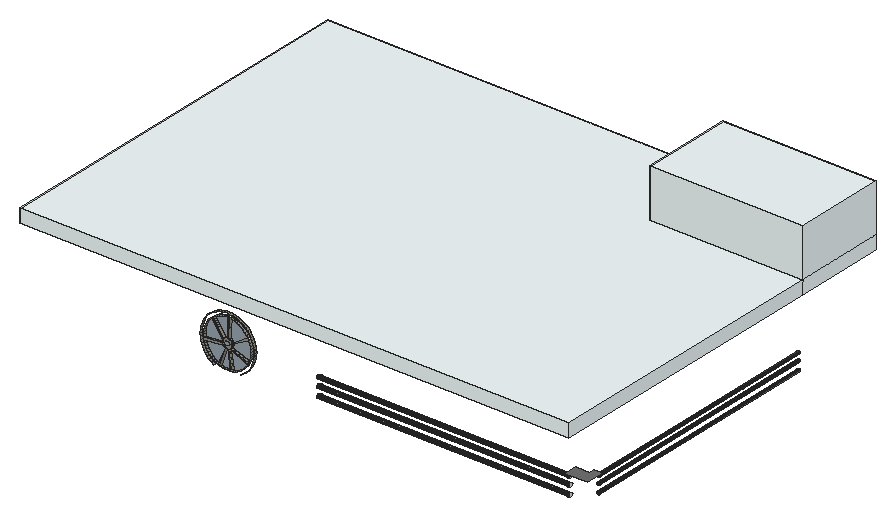
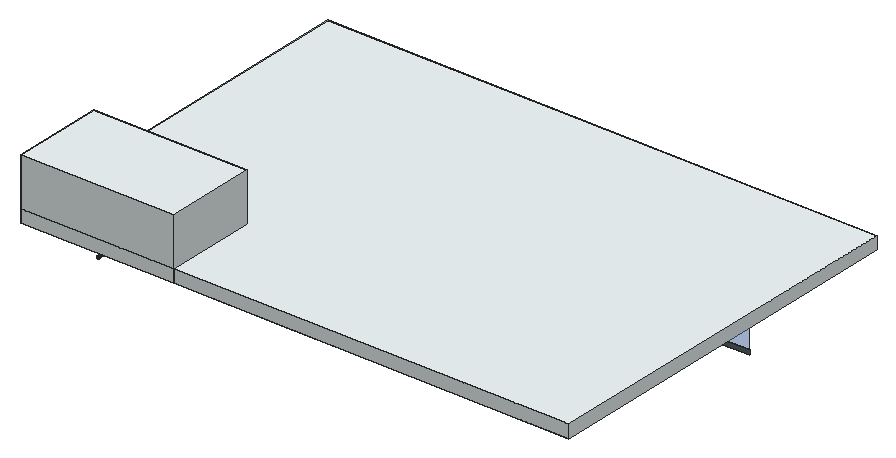
# SketchUp Ruby script. Lengths in inches.
U = 1.inch
M = Sketchup.active_model
def pt(a) = Geom::Point3d.new(a.map { |v| v * U })
def face(e, loops, mat)
  f = e.add_face(loops[0].map { |a| pt(a) })
  loops[1..].each { |l| e.add_face(l.map { |a| pt(a) }).erase! }
  f.material = f.back_material = mat if mat
  f
end
# faces: each face lists its corners as indices into pts; further lists are holes
def faces(e, pts, list, mat = nil) = list.each { |f| face(e, (f[0].is_a?(Array) ? f : [f]).map { |l| l.map { |i| pts[i] } }, mat) }
# xy, xz, yz: faces in a plane at the given z, y or x. An outline is a flat list of corners, or four numbers for a rectangle; further outlines are holes
def ring(l) = l.size == 4 ? [[l[0], l[1]], [l[2], l[1]], [l[2], l[3]], [l[0], l[3]]] : l.each_slice(2).to_a
def flat(e, list, mat, &to3) = list.each { |f| face(e, (f[0].is_a?(Array) ? f : [f]).map { |l| ring(l).map { |u, v| to3.(u, v) } }, mat) }
def xy(e, z, list, mat = nil) = flat(e, list, mat) { |x, y| [x, y, z] }
def xz(e, y, list, mat = nil) = flat(e, list, mat) { |x, z| [x, y, z] }
def yz(e, x, list, mat = nil) = flat(e, list, mat) { |y, z| [x, y, z] }
def lines(e, pts, list) = list.each { |a, b| e.add_line(pt(pts[a]), pt(pts[b])) }
# prism: a flat outline (further loops are holes) pulled along v
def prism(e, loops, v, mat = nil)
  f = face(e, loops, mat); d = Geom::Vector3d.new(v.map { |x| x * U })
  f.pushpull(f.normal.samedirection?(d) ? d.length : -d.length)
end
def box(e, o, s, mat = nil) = prism(e, [[o, [o[0] + s[0], o[1], o[2]], [o[0] + s[0], o[1] + s[1], o[2]], [o[0], o[1] + s[1], o[2]]]], [0, 0, s[2]], mat)
def at(x, y, z, deg = 0) = Geom::Transformation.translation(pt([x, y, z])) * Geom::Transformation.rotation(ORIGIN, Z_AXIS, deg.degrees)
def axes(o, x, y, z) = Geom::Transformation.new([*x, 0, *y, 0, *z, 0, *pt(o).to_a, 1])
def part(name) = M.definitions.add(name)
# library, detail: a bought-in or finely detailed component or shape, given as its bounding box
def library(name, o, s) = part(name).tap { |d| box(d.entities, o, s) }
def detail(e, o, s) = box(e.add_group.entities, o, s)
def put(e, d, t, mat = nil) = e.add_instance(d, t).tap { |i| i.material = mat if mat }
def group(e, t, mat = nil) = e.add_group.tap { |g| g.transformation = t; g.material = mat if mat }.entities
root = M.entities
M.materials.add("[Color M04]").color = [142, 142, 142]
M.materials.add("[Color M05]").color = [114, 114, 114]
M.materials.add("[Formica Graystone]1").color = [149, 146, 135]
M.materials.add("[Formica Speckled Grey]").color = [94, 105, 111]
M.materials.add("[Terrazzo Light Blue]").color = [151, 165, 175]
M.materials.add("[Terrazzo Light Blue]1").color = [196, 214, 227]
M.materials.add("[Translucent Glass Blue]").color = [100, 149, 237]
M.materials["[Translucent Glass Blue]"].alpha = 0.5
M.materials.add("[White Subway Tile]").color = [243, 252, 253]
xy(root,2160.625,[[2109.83,824.72,2111.95,824.99,2113.93,825.8125,2115.625,827.11,2116.92,828.81,2117.74,830.78,2118.02,832.9,2117.74,835.02,2116.92,837,2115.625,838.69,2113.93,839.99,2111.95,840.8125,2109.83,841.09,2107.72,840.8125,2105.74,839.99,2104.04,838.69,2102.74,837,2101.93,835.02,2101.65,832.9,2101.93,830.78,2102.74,828.81,2104.04,827.11,2105.74,825.8125,2107.72,824.99]])
xy(root,2167.3125,[[2949.99,1696.19,2952.05,1696.46,2953.96,1697.25,2955.6,1698.51,2956.87,1700.16,2957.66,1702.07,2957.93,1704.13,2957.66,1706.18,2956.87,1708.1,2955.6,1709.74,2953.96,1711,2952.05,1711.79,2949.99,1712.06,2947.9375,1711.79,2946.02,1711,2944.38,1709.74,2943.12,1708.1,2942.32,1706.18,2942.05,1704.13,2942.32,1702.07,2943.12,1700.16,2944.38,1698.51,2946.02,1697.25,2947.9375,1696.46]])
xy(root,2167.625,[[2949.99,1302.69,2952.05,1302.96,2953.96,1303.75,2955.6,1305.01,2956.87,1306.66,2957.66,1308.57,2957.93,1310.63,2957.66,1312.68,2956.87,1314.6,2955.6,1316.24,2953.96,1317.5,2952.05,1318.29,2949.99,1318.56,2947.9375,1318.29,2946.02,1317.5,2944.38,1316.24,2943.12,1314.6,2942.32,1312.68,2942.05,1310.63,2942.32,1308.57,2943.12,1306.66,2944.38,1305.01,2946.02,1303.75,2947.9375,1302.96]])
xy(root,2183.75,[[2867.16,803.71,2968.68,803.71,2968.68,888.17,2929.99,888.17,2929.99,862.88,2867.16,862.88]],"[Color M05]")
xy(root,2330.11,[[1687.83,876.99,1720.33,1103.3]],"[Terrazzo Light Blue]")
xy(root,2340.5,[[605.8,1146.14,928.48,1221.7]])
xy(root,2410.6875,[[477.43,697.64,547.35,1118.14],[2764.79,697.64,2968.68,2026.57],[1034.97,803.71,1720.33,2026.57],[477.43,1118.14,547.35,1118.14,547.35,1146.14,1034.97,1146.14,1034.97,2026.57,477.43,2026.57],[1720.33,1239.01,2764.79,2026.57],
  [477.43,2026.57,1034.97,2442.87],[1034.97,2026.57,1720.33,2442.87],[1720.33,2026.57,2273.77,2442.87],[2273.77,2026.57,2968.68,2442.87]])
xy(root,2410.6875,[[547.35,697.64,1034.97,1146.14],[1034.97,697.64,1720.33,803.71],[[1720.33,697.64,2764.79,1239.01],[2267.4,882.09,2324.97,939.65]]],"[Terrazzo Light Blue]1")
xy(root,2470.25,[[477.43,697.64,2968.68,2442.87]],"[White Subway Tile]")
xy(root,2688.875,[[2273.77,2026.57,2968.68,2442.87]],"[White Subway Tile]")
xz(root,697.64,[[477.43,2410.6875,2968.68,2470.25]],"[White Subway Tile]")
xz(root,793.39,[[1352.48,2073.62,1363.66,2075.39,1346.76,2160.28],[1307.78,2078.32,1335.6,2160.28,1297.22,2082.37],[1434.79,2127.07,1439.92,2137.15,1356.43,2165.86],[1235.46,2158.64,1322.51,2170.33,1320.36,2175.53,1233.69,2169.8125],[[1341.18,2159.55,1346.76,2160.28,1351.96,2162.4375,1356.43,2165.86,1359.86,2170.33,1362.01,2175.53,1362.75,2181.11,1362.01,2186.69,1359.86,2191.89,1356.43,2196.36,1351.96,2199.79,1346.76,2201.94,1341.18,2202.67,1335.6,2201.94,1330.4,2199.79,1325.9375,2196.36,1322.51,2191.89,1320.36,2186.69,1319.62,2181.11,1320.36,2175.53,1322.51,2170.33,1325.9375,2165.86,1330.4,2162.4375,1335.6,2160.28],[1341.86,2170.07,1339.11,2170.1,1336.45,2170.84,1334.08,2172.24,1332.15,2174.21,1330.79,2176.62,1330.11,2179.29,1330.14,2182.04,1330.88,2184.7,1332.28,2187.07,1334.25,2189,1336.65,2190.36,1339.32,2191.04,1342.08,2191.02,1344.74,2190.27,1347.11,2188.87,1349.04,2186.9,1350.39,2184.5,1351.08,2181.83,1351.05,2179.07,1350.31,2176.42,1348.91,2174.04,1346.9375,2172.11,1344.54,2170.76]],
  [1362.01,2186.69,1439.92,2225.07,1434.79,2235.15],[1322.51,2191.89,1325.9375,2196.36,1277.65,2268.55,1268.86,2261.43],[1346.76,2201.94,1352.48,2288.6,1341.18,2289.2,1341.18,2202.67]],"[Formica Graystone]1")
xz(root,793.39,[[1341.86,2170.07,1344.54,2170.76,1346.9375,2172.11,1348.91,2174.04,1350.31,2176.42,1351.05,2179.07,1351.08,2181.83,1350.39,2184.5,1349.04,2186.9,1347.11,2188.87,1344.74,2190.27,1342.08,2191.02,1339.32,2191.04,1336.65,2190.36,1334.25,2189,1332.28,2187.07,1330.88,2184.7,1330.14,2182.04,1330.11,2179.29,1330.79,2176.62,1332.15,2174.21,1334.08,2172.24,1336.45,2170.84,1339.11,2170.1]],"[Terrazzo Light Blue]")
xz(root,803.71,[[1341.18,2073.03,1352.48,2073.62,1346.76,2160.28,1341.18,2159.55,1335.6,2160.28,1307.78,2078.32,1318.71,2075.39,1329.89,2073.62],[1363.66,2075.39,1374.58,2078.32,1385.15,2082.37,1395.23,2087.51,1404.71,2093.67,1413.51,2100.79,1421.51,2108.79,1428.625,2117.58,1434.79,2127.07,1356.43,2165.86,1351.96,2162.4375,1346.76,2160.28],[1297.22,2082.37,1335.6,2160.28,1330.4,2162.4375,1325.9375,2165.86,1322.51,2170.33,1235.46,2158.64,1238.39,2147.71,1242.44,2137.15,1247.58,2127.07,1253.74,2117.58,1260.86,2108.79,1268.86,2100.79,1277.65,2093.67,1287.14,2087.51],[1439.92,2137.15,1443.98,2147.71,1446.91,2158.64,1448.68,2169.8125,1449.27,2181.11,1448.68,2192.41,1446.91,2203.58,1443.98,2214.51,1439.92,2225.07,1362.01,2186.69,1362.75,2181.11,1362.01,2175.53,1359.86,2170.33,1356.43,2165.86],[1233.69,2169.8125,1320.36,2175.53,1319.62,2181.11,1320.36,2186.69,1322.51,2191.89,1268.86,2261.43,1260.86,2253.43,1253.74,2244.64,1247.58,2235.15,1242.44,2225.07,1238.39,2214.51,1235.46,2203.58,1233.69,2192.41,1233.1,2181.11],
  [1362.01,2186.69,1434.79,2235.15,1428.625,2244.64,1421.51,2253.43,1413.51,2261.43,1404.71,2268.55,1395.23,2274.72,1385.15,2279.85,1374.58,2283.91,1363.66,2286.84,1352.48,2288.6,1346.76,2201.94,1351.96,2199.79,1356.43,2196.36,1359.86,2191.89],[1325.9375,2196.36,1330.4,2199.79,1335.6,2201.94,1341.18,2202.67,1341.18,2289.2,1329.89,2288.6,1318.71,2286.84,1307.78,2283.91,1297.22,2279.85,1287.14,2274.72,1277.65,2268.55]],"[Terrazzo Light Blue]")
xz(root,888.17,[[2950.45,2090.97,2952.01,2091.18,2953.45,2091.77,2954.7,2092.73,2955.65,2093.97,2956.25,2095.42,2956.45,2096.97,2956.25,2098.52,2955.65,2099.97,2954.7,2101.21,2953.45,2102.17,2952.01,2102.77,2950.45,2102.97,2948.9,2102.77,2947.45,2102.17,2946.21,2101.21,2945.26,2099.97,2944.66,2098.52,2944.45,2096.97,2944.66,2095.42,2945.26,2093.97,2946.21,2092.73,2947.45,2091.77,2948.9,2091.18],[2950.45,2128.53,2952.01,2128.74,2953.45,2129.34,2954.7,2130.29,2955.65,2131.53,2956.25,2132.98,2956.45,2134.53,2956.25,2136.09,2955.65,2137.53,2954.7,2138.78,2953.45,2139.73,2952.01,2140.33,2950.45,2140.53,2948.9,2140.33,2947.45,2139.73,2946.21,2138.78,2945.26,2137.53,2944.66,2136.09,2944.45,2134.53,2944.66,2132.98,2945.26,2131.53,2946.21,2130.29,2947.45,2129.34,2948.9,2128.74],[2950.45,2161.72,2952.01,2161.93,2953.45,2162.52,2954.7,2163.48,2955.65,2164.72,2956.25,2166.17,2956.45,2167.72,2956.25,2169.27,2955.65,2170.72,2954.7,2171.96,2953.45,2172.92,2952.01,2173.52,2950.45,2173.72,2948.9,2173.52,2947.45,2172.92,2946.21,2171.96,2945.26,2170.72,2944.66,2169.27,2944.45,2167.72,2944.66,2166.17,2945.26,2164.72,2946.21,2163.48,2947.45,2162.52,2948.9,2161.93]])
xz(root,1221.7,[[631.45,2158.7,755.72,2178.96],[755.72,2158.7,770.95,2178.96],[770.95,2158.7,902.82,2178.96],[755.72,2178.96,770.95,2314.84]],"[Formica Speckled Grey]")
xz(root,1221.7,[[631.45,2178.96,755.72,2314.84],[770.95,2178.96,902.82,2314.84]],"[Translucent Glass Blue]")
xz(root,2026.57,[[2273.77,2410.6875,2968.68,2688.875]],"[White Subway Tile]")
xz(root,2442.87,[[477.43,2410.6875,2273.77,2470.25],[2273.77,2410.6875,2968.68,2470.25],[2273.77,2470.25,2968.68,2688.875]],"[White Subway Tile]")
yz(root,477.43,[[697.64,2410.6875,2442.87,2470.25]],"[White Subway Tile]")
yz(root,1341.18,[[793.39,2202.67,803.71,2289.2]],"[Formica Graystone]1")
yz(root,2273.77,[[2026.57,2410.6875,2442.87,2688.875]],"[White Subway Tile]")
yz(root,2867.16,[[836.16,2075.23,838.2,2075.5,840.1,2076.28,841.73,2077.53,842.98,2079.16,843.77,2081.0625,844.04,2083.1,843.77,2085.14,842.98,2087.04,841.73,2088.67,840.1,2089.92,838.2,2090.71,836.16,2090.98,834.125,2090.71,832.22,2089.92,830.59,2088.67,829.34,2087.04,828.55,2085.14,828.29,2083.1,828.55,2081.0625,829.34,2079.16,830.59,2077.53,832.22,2076.28,834.125,2075.5],[836.16,2115.79,838.2,2116.06,840.1,2116.84,841.73,2118.1,842.98,2119.73,843.77,2121.625,844.04,2123.66,843.77,2125.7,842.98,2127.6,841.73,2129.23,840.1,2130.48,838.2,2131.27,836.16,2131.54,834.125,2131.27,832.22,2130.48,830.59,2129.23,829.34,2127.6,828.55,2125.7,828.29,2123.66,828.55,2121.625,829.34,2119.73,830.59,2118.1,832.22,2116.84,834.125,2116.06],[836.16,2153.1,838.2,2153.37,840.1,2154.16,841.73,2155.41,842.98,2157.04,843.77,2158.9375,844.04,2160.98,843.77,2163.02,842.98,2164.91,841.73,2166.55,840.1,2167.8,838.2,2168.58,836.16,2168.85,834.125,2168.58,832.22,2167.8,830.59,2166.55,829.34,2164.91,828.55,2163.02,828.29,2160.98,828.55,2158.9375,829.34,2157.04,830.59,2155.41,832.22,2154.16,834.125,2153.37]])
yz(root,2968.68,[[697.64,2410.6875,2026.57,2470.25],[2026.57,2410.6875,2442.87,2470.25],[2026.57,2470.25,2442.87,2688.875]],"[White Subway Tile]")
p = [[1341.18,803.71,2073.03],[1329.89,803.71,2073.62],[1329.89,793.39,2073.62],[1341.18,793.39,2073.03],[1352.48,803.71,2073.62],[1352.48,793.39,2073.62],
  [1318.71,803.71,2075.39],[1318.71,793.39,2075.39],[1346.76,803.71,2160.28],[1346.76,793.39,2160.28],[1268.59,803.71,2081.2],[1279.43,803.71,2074.16],
  [1279.43,793.39,2074.16],[1268.59,793.39,2081.2],[1402.93,803.71,2074.16],[1413.77,803.71,2081.2],[1413.77,793.39,2081.2],[1402.93,793.39,2074.16],
  [2867.16,836.16,2075.23],[2867.16,834.125,2075.5],[1720.33,834.125,2075.5],[1720.33,836.16,2075.23],[2867.16,838.2,2075.5],[1720.33,838.2,2075.5],
  [1307.78,803.71,2078.32],[1307.78,793.39,2078.32],[1363.66,803.71,2075.39],[1363.66,793.39,2075.39],[1374.58,803.71,2078.32],[1374.58,793.39,2078.32],
  [2867.16,832.22,2076.28],[1720.33,832.22,2076.28],[2867.16,840.1,2076.28],[1720.33,840.1,2076.28],[2867.16,830.59,2077.53],[1720.33,830.59,2077.53],
  [2867.16,841.73,2077.53],[1720.33,841.73,2077.53],[2867.16,829.34,2079.16],[1720.33,829.34,2079.16],[2867.16,842.98,2079.16],[1720.33,842.98,2079.16],
  [1335.6,803.71,2160.28],[1335.6,793.39,2160.28],[1385.15,803.71,2082.37],[1385.15,793.39,2082.37],[2867.16,828.55,2081.0625],[1720.33,828.55,2081.0625],
  [2867.16,843.77,2081.0625],[1720.33,843.77,2081.0625],[2867.16,828.29,2083.1],[1720.33,828.29,2083.1],[2867.16,844.04,2083.1],[1720.33,844.04,2083.1],
  [1258.55,803.71,2089.33],[1258.55,793.39,2089.33],[1423.82,803.71,2089.33],[1423.82,793.39,2089.33],[1297.22,803.71,2082.37],[1287.14,803.71,2087.51],
  [1287.14,793.39,2087.51],[1297.22,793.39,2082.37],[1395.23,803.71,2087.51],[1395.23,793.39,2087.51],[2867.16,828.55,2085.14],[1720.33,828.55,2085.14],
  [2867.16,843.77,2085.14],[1720.33,843.77,2085.14],[2867.16,829.34,2087.04],[1720.33,829.34,2087.04],[2867.16,842.98,2087.04],[1720.33,842.98,2087.04],
  [2867.16,830.59,2088.67],[1720.33,830.59,2088.67],[2867.16,841.73,2088.67],[1720.33,841.73,2088.67],[1277.65,803.71,2093.67],[1277.65,793.39,2093.67],
  [1404.71,803.71,2093.67],[1404.71,793.39,2093.67],[2867.16,832.22,2089.92],[1720.33,832.22,2089.92],[2867.16,840.1,2089.92],[1720.33,840.1,2089.92],
  [1249.4,803.71,2098.47],[1249.4,793.39,2098.47],[1432.96,803.71,2098.47],[1432.96,793.39,2098.47],[2867.16,834.125,2090.71],[1720.33,834.125,2090.71],
  [2867.16,838.2,2090.71],[1720.33,838.2,2090.71],[2867.16,836.16,2090.98],[1720.33,836.16,2090.98],[2950.45,888.17,2090.97],[2948.9,888.17,2091.18],
  [2948.9,2026.57,2091.18],[2950.45,2026.57,2090.97],[2952.01,888.17,2091.18],[2952.01,2026.57,2091.18],[2947.45,888.17,2091.77],[2947.45,2026.57,2091.77],
  [2953.45,888.17,2091.77],[2953.45,2026.57,2091.77],[2946.21,888.17,2092.73],[2946.21,2026.57,2092.73],[2954.7,888.17,2092.73],[2954.7,2026.57,2092.73],
  [2945.26,888.17,2093.97],[2945.26,2026.57,2093.97],[2955.65,888.17,2093.97],[2955.65,2026.57,2093.97],[1268.86,803.71,2100.79],[1268.86,793.39,2100.79],
  [1413.51,803.71,2100.79],[1413.51,793.39,2100.79],[2944.66,888.17,2095.42],[2944.66,2026.57,2095.42],[2956.25,888.17,2095.42],[2956.25,2026.57,2095.42],
  [2944.45,888.17,2096.97],[2944.45,2026.57,2096.97],[2956.45,888.17,2096.97],[2956.45,2026.57,2096.97],[2944.66,888.17,2098.52],[2944.66,2026.57,2098.52],
  [2956.25,888.17,2098.52],[2956.25,2026.57,2098.52],[1241.27,803.71,2108.52],[1241.27,793.39,2108.52],[1441.1,803.71,2108.52],[1441.1,793.39,2108.52],
  [2945.26,888.17,2099.97],[2945.26,2026.57,2099.97],[2955.65,888.17,2099.97],[2955.65,2026.57,2099.97],[2946.21,888.17,2101.21],[2946.21,2026.57,2101.21],
  [2954.7,888.17,2101.21],[2954.7,2026.57,2101.21],[1260.86,803.71,2108.79],[1260.86,793.39,2108.79],[1421.51,803.71,2108.79],[1421.51,793.39,2108.79],
  [2947.45,888.17,2102.17],[2947.45,2026.57,2102.17],[2953.45,888.17,2102.17],[2953.45,2026.57,2102.17],[2948.9,888.17,2102.77],[2948.9,2026.57,2102.77],
  [2952.01,888.17,2102.77],[2952.01,2026.57,2102.77],[2950.45,888.17,2102.97],[2950.45,2026.57,2102.97],[1234.23,803.71,2119.36],[1234.23,793.39,2119.36],
  [1448.14,803.71,2119.36],[1448.14,793.39,2119.36],[1253.74,803.71,2117.58],[1253.74,793.39,2117.58],[1428.625,803.71,2117.58],[1428.625,793.39,2117.58],
  [2867.16,836.16,2115.79],[2867.16,834.125,2116.06],[1720.33,834.125,2116.06],[1720.33,836.16,2115.79],[2867.16,838.2,2116.06],[1720.33,838.2,2116.06],
  [2867.16,832.22,2116.84],[1720.33,832.22,2116.84],[2867.16,840.1,2116.84],[1720.33,840.1,2116.84],[2867.16,830.59,2118.1],[1720.33,830.59,2118.1],
  [2867.16,841.73,2118.1],[1720.33,841.73,2118.1],[1247.58,803.71,2127.07],[1247.58,793.39,2127.07],[1434.79,803.71,2127.07],[1434.79,793.39,2127.07],
  [2867.16,829.34,2119.73],[1720.33,829.34,2119.73],[2867.16,842.98,2119.73],[1720.33,842.98,2119.73],[1228.36,803.71,2130.88],[1228.36,793.39,2130.88],
  [1454.01,803.71,2130.88],[1454.01,793.39,2130.88],[2867.16,828.55,2121.625],[1720.33,828.55,2121.625],[2867.16,843.77,2121.625],[1720.33,843.77,2121.625],
  [2867.16,828.29,2123.66],[1720.33,828.29,2123.66],[2867.16,844.04,2123.66],[1720.33,844.04,2123.66],[2867.16,828.55,2125.7],[1720.33,828.55,2125.7],
  [2867.16,843.77,2125.7],[1720.33,843.77,2125.7],[2867.16,829.34,2127.6],[1720.33,829.34,2127.6],[2867.16,842.98,2127.6],[1720.33,842.98,2127.6],
  [1242.44,803.71,2137.15],[1242.44,793.39,2137.15],[1356.43,803.71,2165.86],[1356.43,793.39,2165.86],[2867.16,830.59,2129.23],[1720.33,830.59,2129.23],
  [2867.16,841.73,2129.23],[1720.33,841.73,2129.23],[2950.45,888.17,2128.53],[2948.9,888.17,2128.74],[2948.9,2026.57,2128.74],[2950.45,2026.57,2128.53],
  [2952.01,888.17,2128.74],[2952.01,2026.57,2128.74],[2947.45,888.17,2129.34],[2947.45,2026.57,2129.34],[2953.45,888.17,2129.34],[2953.45,2026.57,2129.34],
  [2867.16,832.22,2130.48],[1720.33,832.22,2130.48],[2867.16,840.1,2130.48],[1720.33,840.1,2130.48],[2946.21,888.17,2130.29],[2946.21,2026.57,2130.29],
  [2954.7,888.17,2130.29],[2954.7,2026.57,2130.29],[2945.26,888.17,2131.53],[2945.26,2026.57,2131.53],[2955.65,888.17,2131.53],[2955.65,2026.57,2131.53],
  [2867.16,834.125,2131.27],[1720.33,834.125,2131.27],[2867.16,838.2,2131.27],[1720.33,838.2,2131.27],[1223.73,803.71,2142.95],[1223.73,793.39,2142.95],
  [1458.64,803.71,2142.95],[1458.64,793.39,2142.95],[2867.16,836.16,2131.54],[1720.33,836.16,2131.54],[2944.66,888.17,2132.98],[2944.66,2026.57,2132.98],
  [2956.25,888.17,2132.98],[2956.25,2026.57,2132.98],[2944.45,888.17,2134.53],[2944.45,2026.57,2134.53],[2956.45,888.17,2134.53],[2956.45,2026.57,2134.53],
  [2944.66,888.17,2136.09],[2944.66,2026.57,2136.09],[2956.25,888.17,2136.09],[2956.25,2026.57,2136.09],[2945.26,888.17,2137.53],[2945.26,2026.57,2137.53],
  [2955.65,888.17,2137.53],[2955.65,2026.57,2137.53],[1238.39,803.71,2147.71],[1238.39,793.39,2147.71],[1439.92,803.71,2137.15],[1439.92,793.39,2137.15],
  [1443.98,803.71,2147.71],[1443.98,793.39,2147.71],[2946.21,888.17,2138.78],[2946.21,2026.57,2138.78],[2954.7,888.17,2138.78],[2954.7,2026.57,2138.78],
  [2947.45,888.17,2139.73],[2947.45,2026.57,2139.73],[2953.45,888.17,2139.73],[2953.45,2026.57,2139.73],[2948.9,888.17,2140.33],[2948.9,2026.57,2140.33],
  [2952.01,888.17,2140.33],[2952.01,2026.57,2140.33],[2950.45,888.17,2140.53],[2950.45,2026.57,2140.53],[1220.38,803.71,2155.43],[1220.38,793.39,2155.43],
  [1461.98,803.71,2155.43],[1461.98,793.39,2155.43],[1235.46,803.71,2158.64],[1235.46,793.39,2158.64],[1446.91,803.71,2158.64],[1446.91,793.39,2158.64],
  [2867.16,836.16,2153.1],[2867.16,834.125,2153.37],[1720.33,834.125,2153.37],[1720.33,836.16,2153.1],[2867.16,838.2,2153.37],[1720.33,838.2,2153.37],
  [2867.16,832.22,2154.16],[1720.33,832.22,2154.16],[2867.16,840.1,2154.16],[1720.33,840.1,2154.16],[2867.16,830.59,2155.41],[1720.33,830.59,2155.41],
  [2867.16,841.73,2155.41],[1720.33,841.73,2155.41],[1218.36,803.71,2168.2],[1218.36,793.39,2168.2],[1464.01,803.71,2168.2],[1464.01,793.39,2168.2],
  [2867.16,829.34,2157.04],[1720.33,829.34,2157.04],[2867.16,842.98,2157.04],[1720.33,842.98,2157.04],[2867.16,828.55,2158.9375],[1720.33,828.55,2158.9375],
  [2867.16,843.77,2158.9375],[1720.33,843.77,2158.9375],[1322.51,803.71,2170.33],[1322.51,793.39,2170.33],[1448.68,803.71,2169.8125],[1448.68,793.39,2169.8125],
  [2867.16,828.29,2160.98],[1720.33,828.29,2160.98],[2867.16,844.04,2160.98],[1720.33,844.04,2160.98],[1341.18,803.71,2159.55],[1341.18,793.39,2159.55],
  [1330.4,803.71,2162.4375],[1330.4,793.39,2162.4375],[1351.96,803.71,2162.4375],[1351.96,793.39,2162.4375],[2867.16,828.55,2163.02],[1720.33,828.55,2163.02],
  [2867.16,843.77,2163.02],[1720.33,843.77,2163.02],[2950.45,888.17,2161.72],[2948.9,888.17,2161.93],[2948.9,2026.57,2161.93],[2950.45,2026.57,2161.72],
  [2952.01,888.17,2161.93],[2952.01,2026.57,2161.93],[2947.45,888.17,2162.52],[2947.45,2026.57,2162.52],[2953.45,888.17,2162.52],[2953.45,2026.57,2162.52],
  [1325.9375,803.71,2165.86],[1325.9375,793.39,2165.86],[2946.21,888.17,2163.48],[2946.21,2026.57,2163.48],[2954.7,888.17,2163.48],[2954.7,2026.57,2163.48],
  [2867.16,829.34,2164.91],[1720.33,829.34,2164.91],[2867.16,842.98,2164.91],[1720.33,842.98,2164.91],[2945.26,888.17,2164.72],[2945.26,2026.57,2164.72],
  [2955.65,888.17,2164.72],[2955.65,2026.57,2164.72],[2944.66,888.17,2166.17],[2944.66,2026.57,2166.17],[2956.25,888.17,2166.17],[2956.25,2026.57,2166.17],
  [2867.16,830.59,2166.55],[1720.33,830.59,2166.55],[2867.16,841.73,2166.55],[1720.33,841.73,2166.55],[1359.86,803.71,2170.33],[1359.86,793.39,2170.33],
  [2944.45,888.17,2167.72],[2944.45,2026.57,2167.72],[2956.45,888.17,2167.72],[2956.45,2026.57,2167.72],[2867.16,832.22,2167.8],[1720.33,832.22,2167.8],
  [2867.16,840.1,2167.8],[1720.33,840.1,2167.8],[2944.66,888.17,2169.27],[2944.66,2026.57,2169.27],[2956.25,888.17,2169.27],[2956.25,2026.57,2169.27],
  [2867.16,834.125,2168.58],[1720.33,834.125,2168.58],[2867.16,838.2,2168.58],[1720.33,838.2,2168.58],[1217.68,803.71,2181.11],[1217.68,793.39,2181.11],
  [1464.68,803.71,2181.11],[1464.68,793.39,2181.11],[2867.16,836.16,2168.85],[1720.33,836.16,2168.85],[2945.26,888.17,2170.72],[2945.26,2026.57,2170.72],
  [2955.65,888.17,2170.72],[2955.65,2026.57,2170.72],[1233.69,803.71,2169.8125],[1233.1,803.71,2181.11],[1233.1,793.39,2181.11],[1233.69,793.39,2169.8125],
  [1320.36,803.71,2175.53],[1320.36,793.39,2175.53],[1449.27,803.71,2181.11],[1449.27,793.39,2181.11],[1362.01,803.71,2175.53],[1362.01,793.39,2175.53],
  [2946.21,888.17,2171.96],[2946.21,2026.57,2171.96],[2954.7,888.17,2171.96],[2954.7,2026.57,2171.96],[2947.45,888.17,2172.92],[2947.45,2026.57,2172.92],
  [2953.45,888.17,2172.92],[2953.45,2026.57,2172.92],[2948.9,888.17,2173.52],[2948.9,2026.57,2173.52],[2952.01,888.17,2173.52],[2952.01,2026.57,2173.52],
  [2950.45,888.17,2173.72],[2950.45,2026.57,2173.72],[1319.62,803.71,2181.11],[1319.62,793.39,2181.11],[1362.75,803.71,2181.11],[1362.75,793.39,2181.11],
  [1218.36,803.71,2194.02],[1218.36,793.39,2194.02],[1233.69,803.71,2192.41],[1233.69,793.39,2192.41],[1320.36,803.71,2186.69],[1320.36,793.39,2186.69],
  [1362.01,803.71,2186.69],[1362.01,793.39,2186.69],[1448.68,803.71,2192.41],[1448.68,793.39,2192.41],[1464.01,803.71,2194.02],[1464.01,793.39,2194.02],
  [1322.51,803.71,2191.89],[1322.51,793.39,2191.89],[1359.86,803.71,2191.89],[1359.86,793.39,2191.89],[1434.79,803.71,2235.15],[1434.79,793.39,2235.15],
  [1439.92,803.71,2225.07],[1439.92,793.39,2225.07],[1268.86,803.71,2261.43],[1268.86,793.39,2261.43],[1356.43,803.71,2196.36],[1356.43,793.39,2196.36],
  [1235.46,803.71,2203.58],[1235.46,793.39,2203.58],[1446.91,803.71,2203.58],[1446.91,793.39,2203.58],[1220.38,803.71,2206.79],[1220.38,793.39,2206.79],
  [1461.98,803.71,2206.79],[1461.98,793.39,2206.79],[1325.9375,803.71,2196.36],[1277.65,803.71,2268.55],[1277.65,793.39,2268.55],[1325.9375,793.39,2196.36],
  [1330.4,803.71,2199.79],[1330.4,793.39,2199.79],[1351.96,803.71,2199.79],[1351.96,793.39,2199.79],[1335.6,803.71,2201.94],[1335.6,793.39,2201.94],
  [1346.76,803.71,2201.94],[1346.76,793.39,2201.94],[1341.18,803.71,2202.67],[1341.18,793.39,2202.67],[1352.48,803.71,2288.6],[1352.48,793.39,2288.6],
  [1238.39,803.71,2214.51],[1238.39,793.39,2214.51],[1443.98,803.71,2214.51],[1443.98,793.39,2214.51],[1223.73,803.71,2219.28],[1223.73,793.39,2219.28],
  [1458.64,803.71,2219.28],[1458.64,793.39,2219.28],[1242.44,803.71,2225.07],[1242.44,793.39,2225.07],[1228.36,803.71,2231.34],[1228.36,793.39,2231.34],
  [1454.01,803.71,2231.34],[1454.01,793.39,2231.34],[1247.58,803.71,2235.15],[1247.58,793.39,2235.15],[1234.23,803.71,2242.86],[1234.23,793.39,2242.86],
  [1448.14,803.71,2242.86],[1448.14,793.39,2242.86],[1253.74,803.71,2244.64],[1253.74,793.39,2244.64],[1428.625,803.71,2244.64],[1428.625,793.39,2244.64],
  [1241.27,803.71,2253.7],[1241.27,793.39,2253.7],[1441.1,803.71,2253.7],[1441.1,793.39,2253.7],[1260.86,803.71,2253.43],[1260.86,793.39,2253.43],
  [1421.51,803.71,2253.43],[1421.51,793.39,2253.43],[1413.51,803.71,2261.43],[1413.51,793.39,2261.43],[1249.4,803.71,2263.75],[1249.4,793.39,2263.75],
  [1432.96,803.71,2263.75],[1432.96,793.39,2263.75],[1404.71,803.71,2268.55],[1404.71,793.39,2268.55],[1258.55,803.71,2272.89],[1258.55,793.39,2272.89],
  [1423.82,803.71,2272.89],[1423.82,793.39,2272.89],[1287.14,803.71,2274.72],[1287.14,793.39,2274.72],[1395.23,803.71,2274.72],[1395.23,793.39,2274.72],
  [1268.59,803.71,2281.03],[1268.59,793.39,2281.03],[1413.77,803.71,2281.03],[1413.77,793.39,2281.03],[1297.22,803.71,2279.85],[1297.22,793.39,2279.85],
  [1385.15,803.71,2279.85],[1385.15,793.39,2279.85],[1307.78,803.71,2283.91],[1307.78,793.39,2283.91],[1374.58,803.71,2283.91],[1374.58,793.39,2283.91],
  [1279.43,803.71,2288.07],[1279.43,793.39,2288.07],[1402.93,803.71,2288.07],[1402.93,793.39,2288.07],[1318.71,803.71,2286.84],[1318.71,793.39,2286.84],
  [1363.66,803.71,2286.84],[1363.66,793.39,2286.84],[1329.89,803.71,2288.6],[1329.89,793.39,2288.6],[1290.95,803.71,2293.93],[1290.95,793.39,2293.93],
  [1391.42,803.71,2293.93],[1391.42,793.39,2293.93],[1341.18,803.71,2289.2],[1341.18,793.39,2289.2],[1303.02,803.71,2298.57],[1303.02,793.39,2298.57],
  [1379.35,803.71,2298.57],[1379.35,793.39,2298.57],[1315.51,803.71,2301.91],[1315.51,793.39,2301.91],[1366.86,803.71,2301.91],[1366.86,793.39,2301.91],
  [1328.27,803.71,2303.94],[1328.27,793.39,2303.94],[1354.09,803.71,2303.94],[1354.09,793.39,2303.94],[1341.18,803.71,2304.61],[1341.18,793.39,2304.61]]
faces(root,p,[[0,1,2,3],[4,0,3,5],[1,6,7,2],[8,4,5,9],[10,11,12,13],[14,15,16,17],[6,24,25,7],[26,8,9,27],
  [28,26,27,29],[24,42,43,25],[44,28,29,45],[54,10,13,55],[15,56,57,16],[58,59,60,61],[42,58,61,43],[62,44,45,63],
  [59,76,77,60],[78,62,63,79],[84,54,55,85],[56,86,87,57],[76,112,113,77],[114,78,79,115],[128,84,85,129],[86,130,131,87],
  [112,140,141,113],[142,114,115,143],[154,128,129,155],[130,156,157,131],[140,158,159,141],[160,142,143,161],[158,176,177,159],[178,160,161,179],
  [184,154,155,185],[156,186,187,157],[176,204,205,177],[206,178,179,207],[238,184,185,239],[186,240,241,187],[204,260,261,205],[262,206,207,263],
  [264,262,263,265],[280,238,239,281],[240,282,283,241],[260,284,285,261],[286,264,265,287],[302,280,281,303],[282,304,305,283],[284,314,315,285],
  [316,286,287,317],[42,322,323,43],[322,8,9,323],[324,42,43,325],[8,326,327,9],[342,324,325,343],[326,206,207,327],[314,342,343,315],
  [206,364,365,207],[382,302,303,383],[304,384,385,305],[392,393,394,395],[396,392,395,397],[398,316,317,399],[364,400,401,365],[416,396,397,417],
  [400,418,419,401],[420,382,383,421],[393,422,423,394],[424,416,417,425],[418,426,427,419],[428,398,399,429],[384,430,431,385],[432,424,425,433],
  [426,434,435,427],[436,426,427,437],[426,438,439,427],[440,432,433,441],[434,442,443,435],[422,444,445,423],[446,428,429,447],[448,420,421,449],
  [430,450,451,431],[452,453,454,455],[456,452,455,457],[442,458,459,443],[460,456,457,461],[458,462,463,459],[464,460,461,465],[462,466,467,463],
  [444,468,469,445],[470,446,447,471],[472,448,449,473],[450,474,475,451],[468,476,477,469],[438,470,471,439],[478,472,473,479],[474,480,481,475],
  [476,482,483,477],[484,478,479,485],[480,486,487,481],[482,488,489,483],[490,436,437,491],[492,484,485,493],[486,494,495,487],[488,496,497,489],
  [498,490,491,499],[496,440,441,497],[500,498,499,501],[502,492,493,503],[494,504,505,495],[506,500,501,507],[508,502,503,509],[504,510,511,505],
  [453,512,513,454],[514,506,507,515],[516,508,509,517],[510,518,519,511],[512,520,521,513],[522,514,515,523],[520,524,525,521],[526,522,523,527],
  [528,516,517,529],[518,530,531,519],[524,532,533,525],[534,526,527,535],[532,536,537,533],[466,534,535,467],[538,528,529,539],[530,540,541,531],
  [536,542,543,537],[544,538,539,545],[540,546,547,541],[548,544,545,549],[546,550,551,547],[552,548,549,553],[550,554,555,551],[556,552,553,557],
  [554,556,557,555]],"[Formica Graystone]1")
faces(root,p,[[18,19,20,21],[22,18,21,23],[19,30,31,20],[32,22,23,33],[30,34,35,31],[36,32,33,37],[34,38,39,35],[40,36,37,41],
  [38,46,47,39],[48,40,41,49],[46,50,51,47],[52,48,49,53],[50,64,65,51],[66,52,53,67],[64,68,69,65],[70,66,67,71],
  [68,72,73,69],[74,70,71,75],[72,80,81,73],[82,74,75,83],[80,88,89,81],[90,82,83,91],[88,92,93,89],[92,90,91,93],
  [94,95,96,97],[98,94,97,99],[95,100,101,96],[102,98,99,103],[100,104,105,101],[106,102,103,107],[104,108,109,105],[110,106,107,111],
  [108,116,117,109],[118,110,111,119],[116,120,121,117],[122,118,119,123],[120,124,125,121],[126,122,123,127],[124,132,133,125],[134,126,127,135],
  [132,136,137,133],[138,134,135,139],[136,144,145,137],[146,138,139,147],[144,148,149,145],[150,146,147,151],[148,152,153,149],[152,150,151,153],
  [162,163,164,165],[166,162,165,167],[163,168,169,164],[170,166,167,171],[168,172,173,169],[174,170,171,175],[172,180,181,173],[182,174,175,183],
  [180,188,189,181],[190,182,183,191],[188,192,193,189],[194,190,191,195],[192,196,197,193],[198,194,195,199],[196,200,201,197],[202,198,199,203],
  [200,208,209,201],[210,202,203,211],[212,213,214,215],[216,212,215,217],[213,218,219,214],[220,216,217,221],[208,222,223,209],[224,210,211,225],
  [218,226,227,219],[228,220,221,229],[226,230,231,227],[232,228,229,233],[222,234,235,223],[236,224,225,237],[234,242,243,235],[242,236,237,243],
  [230,244,245,231],[246,232,233,247],[244,248,249,245],[250,246,247,251],[248,252,253,249],[254,250,251,255],[252,256,257,253],[258,254,255,259],
  [256,266,267,257],[268,258,259,269],[266,270,271,267],[272,268,269,273],[270,274,275,271],[276,272,273,277],[274,278,279,275],[278,276,277,279],
  [288,289,290,291],[292,288,291,293],[289,294,295,290],[296,292,293,297],[294,298,299,295],[300,296,297,301],[298,306,307,299],[308,300,301,309],
  [306,310,311,307],[312,308,309,313],[310,318,319,311],[320,312,313,321],[318,328,329,319],[330,320,321,331],[328,348,349,329],[350,330,331,351],
  [348,360,361,349],[362,350,351,363],[360,370,371,361],[372,362,363,373],[370,378,379,371],[380,372,373,381],[378,386,387,379],[386,380,381,387]],"[Color M04]")
faces(root,p,[[332,333,334,335],[336,332,335,337],[333,338,339,334],[340,336,337,341],[338,344,345,339],[346,340,341,347],[344,352,353,345],[354,346,347,355],
  [352,356,357,353],[358,354,355,359],[356,366,367,357],[368,358,359,369],[366,374,375,367],[376,368,369,377],[374,388,389,375],[390,376,377,391],
  [388,402,403,389],[404,390,391,405],[402,406,407,403],[408,404,405,409],[406,410,411,407],[412,408,409,413],[410,414,415,411],[414,412,413,415]],"[Color M05]")
